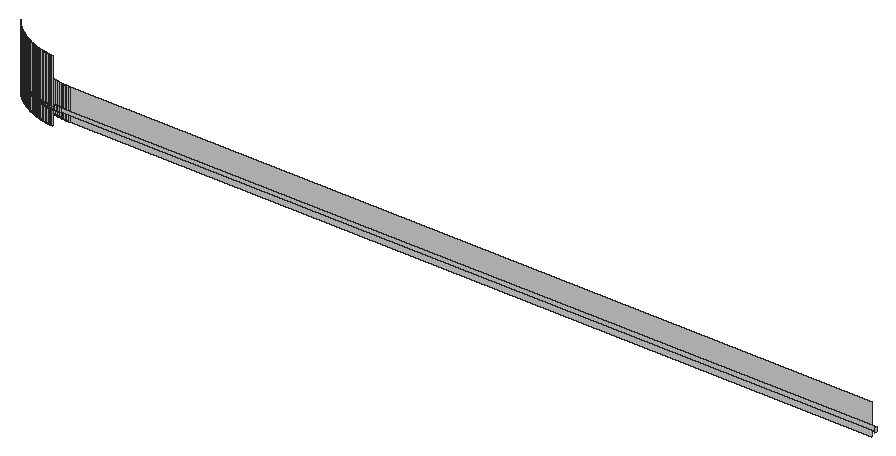
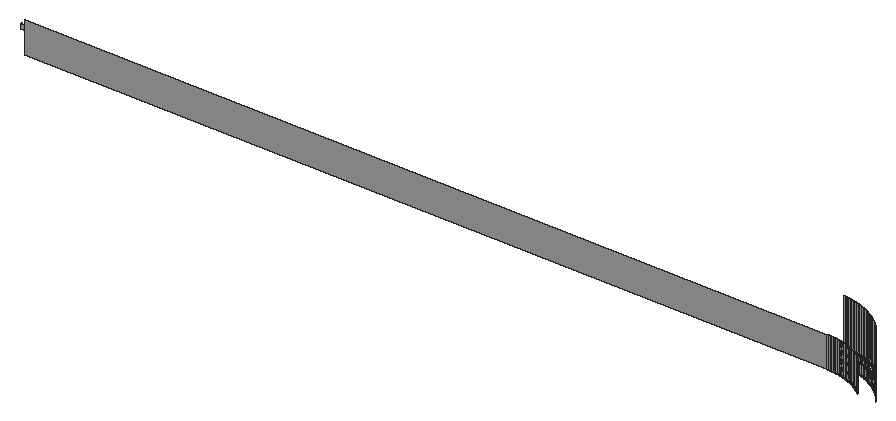
# SketchUp Ruby script. Lengths in inches.
U = 1.inch
M = Sketchup.active_model
def pt(a) = Geom::Point3d.new(a.map { |v| v * U })
def face(e, loops, mat)
  f = e.add_face(loops[0].map { |a| pt(a) })
  loops[1..].each { |l| e.add_face(l.map { |a| pt(a) }).erase! }
  f.material = f.back_material = mat if mat
  f
end
# faces: each face lists its corners as indices into pts; further lists are holes
def faces(e, pts, list, mat = nil) = list.each { |f| face(e, (f[0].is_a?(Array) ? f : [f]).map { |l| l.map { |i| pts[i] } }, mat) }
# xy, xz, yz: faces in a plane at the given z, y or x. An outline is a flat list of corners, or four numbers for a rectangle; further outlines are holes
def ring(l) = l.size == 4 ? [[l[0], l[1]], [l[2], l[1]], [l[2], l[3]], [l[0], l[3]]] : l.each_slice(2).to_a
def flat(e, list, mat, &to3) = list.each { |f| face(e, (f[0].is_a?(Array) ? f : [f]).map { |l| ring(l).map { |u, v| to3.(u, v) } }, mat) }
def xy(e, z, list, mat = nil) = flat(e, list, mat) { |x, y| [x, y, z] }
def xz(e, y, list, mat = nil) = flat(e, list, mat) { |x, z| [x, y, z] }
def yz(e, x, list, mat = nil) = flat(e, list, mat) { |y, z| [x, y, z] }
def lines(e, pts, list) = list.each { |a, b| e.add_line(pt(pts[a]), pt(pts[b])) }
# prism: a flat outline (further loops are holes) pulled along v
def prism(e, loops, v, mat = nil)
  f = face(e, loops, mat); d = Geom::Vector3d.new(v.map { |x| x * U })
  f.pushpull(f.normal.samedirection?(d) ? d.length : -d.length)
end
def box(e, o, s, mat = nil) = prism(e, [[o, [o[0] + s[0], o[1], o[2]], [o[0] + s[0], o[1] + s[1], o[2]], [o[0], o[1] + s[1], o[2]]]], [0, 0, s[2]], mat)
def at(x, y, z, deg = 0) = Geom::Transformation.translation(pt([x, y, z])) * Geom::Transformation.rotation(ORIGIN, Z_AXIS, deg.degrees)
def axes(o, x, y, z) = Geom::Transformation.new([*x, 0, *y, 0, *z, 0, *pt(o).to_a, 1])
def part(name) = M.definitions.add(name)
# library, detail: a bought-in or finely detailed component or shape, given as its bounding box
def library(name, o, s) = part(name).tap { |d| box(d.entities, o, s) }
def detail(e, o, s) = box(e.add_group.entities, o, s)
def put(e, d, t, mat = nil) = e.add_instance(d, t).tap { |i| i.material = mat if mat }
def group(e, t, mat = nil) = e.add_group.tap { |g| g.transformation = t; g.material = mat if mat }.entities
root = M.entities
M.materials.add("[Quartz Light Brown]").color = [215, 212, 212]
xz(root,194.5,[[17.77,114,18,115],[18,114,201,115]],"[Quartz Light Brown]")
xz(root,194.51,[[17.3125,114,17.54,115]],"[Quartz Light Brown]")
xz(root,197,[[17.8,111,18,118],[18,111,198,118]],"[Quartz Light Brown]")
xz(root,197.01,[[17.41,111,17.61,118]],"[Quartz Light Brown]")
yz(root,201,[[194,114,194.5,115]],"[Quartz Light Brown]")
p = [[15.65,194.15,114],[15.65,194.15,111],[15.88,194.125,111],[15.88,194.125,114],[16.12,194.1,111],[16.12,194.1,114],
  [16.35,194.08,111],[16.35,194.08,114],[16.59,194.06,111],[16.59,194.06,114],[14.95,194.26,114],[14.95,194.26,111],
  [15.18,194.22,111],[15.18,194.22,114],[15.42,194.1875,111],[15.42,194.1875,114],[14.26,194.39,114],[14.26,194.39,111],
  [14.49,194.35,111],[14.49,194.35,114],[14.72,194.3,111],[14.72,194.3,114],[13.8,194.5,114],[13.8,194.5,111],
  [14.03,194.44,111],[14.03,194.44,114],[13.57,194.55,114],[13.57,194.55,111],[13.11,194.68,114],[13.11,194.68,111],
  [13.34,194.61,111],[13.34,194.61,114],[12.66,194.81,114],[12.66,194.81,111],[12.89,194.74,111],[12.89,194.74,114],
  [12.4375,194.88,114],[12.4375,194.88,111],[12.21,194.96,114],[12.21,194.96,111],[11.77,195.11,114],[11.77,195.11,111],
  [11.99,195.03,111],[11.99,195.03,114],[11.55,195.2,114],[11.55,195.2,111],[11.33,195.28,114],[11.33,195.28,111],
  [11.11,195.37,114],[11.11,195.37,111],[10.89,195.46,114],[10.89,195.46,111],[10.68,195.56,114],[10.68,195.56,111],
  [10.46,195.65,114],[10.46,195.65,111],[10.25,195.75,114],[10.25,195.75,111],[10.04,195.86,114],[10.04,195.86,111],
  [9.83,195.96,114],[9.83,195.96,111],[9.62,196.07,114],[9.62,196.07,111],[9.41,196.18,114],[9.41,196.18,111],
  [9.2,196.3,114],[9.2,196.3,111],[9,196.41,114],[9,196.41,111],[8.8,196.53,114],[8.8,196.53,111],
  [8.6,196.65,114],[8.6,196.65,111],[8.39,196.78,114],[8.39,196.78,111],[8.2,196.9,114],[8.2,196.9,111],
  [8,197.03,114],[8,197.03,111],[7.8,197.17,114],[7.8,197.17,111],[16.63,197.0625,118],[16.82,197.05,118],
  [16.82,197.05,111],[16.63,197.0625,111],[17.02,197.03,118],[17.02,197.03,111],[17.21,197.02,118],[17.21,197.02,111],
  [17.41,197.01,118],[17.41,197.01,111],[17.61,197.01,118],[17.8,197,118],[17.8,197,111],[17.61,197.01,111],
  [15.85,197.16,118],[16.04,197.13,118],[16.04,197.13,111],[15.85,197.16,111],[16.24,197.1,118],[16.24,197.1,111],
  [16.43,197.08,118],[16.43,197.08,111],[7.61,197.3,114],[7.61,197.3,111],[15.27,197.25,118],[15.46,197.22,118],
  [15.46,197.22,111],[15.27,197.25,111],[15.65,197.18,118],[15.65,197.18,111],[7.42,197.4375,114],[7.42,197.4375,111],
  [14.69,197.37,118],[14.88,197.33,118],[14.88,197.33,111],[14.69,197.37,111],[15.07,197.29,118],[15.07,197.29,111],
  [7.23,197.58,114],[7.23,197.58,111],[14.31,197.46,118],[14.5,197.41,118],[14.5,197.41,111],[14.31,197.46,111],
  [13.93,197.5625,118],[14.12,197.51,118],[14.12,197.51,111],[13.93,197.5625,111],[7.04,197.72,114],[7.04,197.72,111],
  [13.55,197.67,118],[13.74,197.62,118],[13.74,197.62,111],[13.55,197.67,111],[6.86,197.86,114],[6.86,197.86,111],
  [13.18,197.8,118],[13.36,197.73,118],[13.36,197.73,111],[13.18,197.8,111],[12.99,197.86,118],[12.99,197.86,111],
  [6.67,198.01,114],[6.67,198.01,111],[12.625,198,118],[12.81,197.93,118],[12.81,197.93,111],[12.625,198,111],
  [6.49,198.16,114],[6.49,198.16,111],[12.44,198.07,118],[12.44,198.07,111],[12.08,198.22,118],[12.26,198.14,118],
  [12.26,198.14,111],[12.08,198.22,111],[6.31,198.3125,114],[6.31,198.3125,111],[11.9,198.3,118],[11.9,198.3,111],
  [6.13,198.47,114],[6.13,198.47,111],[11.72,198.38,118],[11.72,198.38,111],[11.54,198.46,118],[11.54,198.46,111],
  [5.96,198.625,114],[5.96,198.625,111],[11.19,198.63,118],[11.37,198.55,118],[11.37,198.55,111],[11.19,198.63,111],
  [5.78,198.78,114],[5.78,198.78,111],[11.02,198.73,118],[11.02,198.73,111],[10.84,198.82,118],[10.84,198.82,111],
  [5.61,198.94,114],[5.61,198.94,111],[10.67,198.91,118],[10.67,198.91,111],[5.44,199.11,114],[5.44,199.11,111],
  [10.5,199.01,118],[10.5,199.01,111],[10.33,199.11,118],[10.33,199.11,111],[5.27,199.27,114],[5.27,199.27,111],
  [10.16,199.21,118],[10.16,199.21,111],[10,199.3125,118],[10,199.3125,111],[5.11,199.44,114],[5.11,199.44,111],
  [9.83,199.42,118],[9.83,199.42,111],[4.94,199.61,114],[4.94,199.61,111],[9.67,199.53,118],[9.67,199.53,111],
  [9.5,199.64,118],[9.5,199.64,111],[4.78,199.78,114],[4.78,199.78,111],[9.34,199.75,118],[9.34,199.75,111],
  [4.625,199.96,114],[4.625,199.96,111],[9.18,199.86,118],[9.18,199.86,111],[9.03,199.98,118],[9.03,199.98,111],
  [4.47,200.13,114],[4.47,200.13,111],[8.87,200.1,118],[8.87,200.1,111],[4.3125,200.31,114],[4.3125,200.31,111],
  [8.71,200.22,118],[8.71,200.22,111],[8.56,200.34,118],[8.56,200.34,111],[4.16,200.49,114],[4.16,200.49,111],
  [8.41,200.47,118],[8.41,200.47,111],[4.01,200.67,114],[4.01,200.67,111],[8.26,200.59,118],[8.26,200.59,111],
  [16.625,194.55,115],[16.625,194.55,114],[16.86,194.54,114],[16.86,194.54,115],[17.08,194.52,114],[17.08,194.52,115],
  [17.3125,194.51,114],[17.3125,194.51,115],[17.54,194.51,115],[17.54,194.51,114],[17.77,194.5,114],[17.77,194.5,115],
  [15.49,194.68,115],[15.49,194.68,114],[15.72,194.65,114],[15.72,194.65,115],[15.94,194.62,114],[15.94,194.62,115],
  [16.17,194.6,114],[16.17,194.6,115],[16.4,194.57,114],[16.4,194.57,115],[15.04,194.75,115],[15.04,194.75,114],
  [15.26,194.72,114],[15.26,194.72,115],[14.36,194.88,115],[14.36,194.88,114],[14.59,194.84,114],[14.59,194.84,115],
  [14.8125,194.79,114],[14.8125,194.79,115],[13.91,194.98,115],[13.91,194.98,114],[14.14,194.93,114],[14.14,194.93,115],
  [13.47,195.1,115],[13.47,195.1,114],[13.69,195.04,114],[13.69,195.04,115],[13.25,195.16,115],[13.25,195.16,114],
  [12.8125,195.29,115],[12.8125,195.29,114],[13.03,195.22,114],[13.03,195.22,115],[12.59,195.36,115],[12.59,195.36,114],
  [12.16,195.5,115],[12.16,195.5,114],[12.375,195.43,114],[12.375,195.43,115],[11.94,195.58,115],[11.94,195.58,114],
  [11.73,195.66,115],[11.73,195.66,114],[11.3,195.83,115],[11.3,195.83,114],[11.52,195.75,114],[11.52,195.75,115],
  [11.09,195.92,115],[11.09,195.92,114],[10.88,196.01,115],[10.88,196.01,114],[10.67,196.11,115],[10.67,196.11,114],
  [10.47,196.2,115],[10.47,196.2,114],[10.26,196.3,115],[10.26,196.3,114],[10.06,196.41,115],[10.06,196.41,114],
  [9.85,196.51,115],[9.85,196.51,114],[9.65,196.62,115],[9.65,196.62,114],[9.45,196.73,115],[9.45,196.73,114],
  [9.25,196.84,115],[9.25,196.84,114],[9.05,196.96,115],[9.05,196.96,114],[8.86,197.08,115],[8.86,197.08,114],
  [8.66,197.2,115],[8.66,197.2,114],[8.47,197.32,115],[8.47,197.32,114],[8.28,197.45,115],[8.28,197.45,114],
  [8.09,197.58,115],[8.09,197.58,114],[7.9,197.71,115],[7.9,197.71,114],[7.71,197.84,115],[7.71,197.84,114],
  [7.53,197.98,115],[7.53,197.98,114],[7.35,198.12,115],[7.35,198.12,114],[7.17,198.26,115],[7.17,198.26,114],
  [6.99,198.4,115],[6.99,198.4,114],[6.81,198.55,115],[6.81,198.55,114],[6.63,198.69,115],[6.63,198.69,114],
  [6.46,198.84,115],[6.46,198.84,114],[6.29,198.99,115],[6.29,198.99,114],[6.12,199.15,115],[6.12,199.15,114],
  [5.95,199.31,115],[5.95,199.31,114],[5.79,199.46,115],[5.79,199.46,114],[5.625,199.625,115],[5.625,199.625,114],
  [5.46,199.79,115],[5.46,199.79,114],[5.31,199.95,115],[5.31,199.95,114],[5.15,200.12,115],[5.15,200.12,114],
  [4.99,200.29,115],[4.99,200.29,114],[4.84,200.46,115],[4.84,200.46,114],[4.69,200.63,115],[4.69,200.63,114],
  [15.65,194.15,125],[15.65,194.15,115],[15.88,194.125,115],[15.88,194.125,125],[16.12,194.1,115],[16.12,194.1,125],
  [16.35,194.08,115],[16.35,194.08,125],[16.59,194.06,115],[16.59,194.06,125],[14.95,194.26,125],[14.95,194.26,115],
  [15.18,194.22,115],[15.18,194.22,125],[15.42,194.1875,115],[15.42,194.1875,125],[14.26,194.39,125],[14.26,194.39,115],
  [14.49,194.35,115],[14.49,194.35,125],[14.72,194.3,115],[14.72,194.3,125],[13.8,194.5,125],[13.8,194.5,115],
  [14.03,194.44,115],[14.03,194.44,125],[13.57,194.55,125],[13.57,194.55,115],[13.11,194.68,125],[13.11,194.68,115],
  [13.34,194.61,115],[13.34,194.61,125],[12.66,194.81,125],[12.66,194.81,115],[12.89,194.74,115],[12.89,194.74,125],
  [12.4375,194.88,125],[12.4375,194.88,115],[12.21,194.96,125],[12.21,194.96,115],[11.77,195.11,125],[11.77,195.11,115],
  [11.99,195.03,115],[11.99,195.03,125],[11.55,195.2,125],[11.55,195.2,115],[11.33,195.28,125],[11.33,195.28,115],
  [11.11,195.37,125],[11.11,195.37,115],[10.89,195.46,125],[10.89,195.46,115],[10.68,195.56,125],[10.68,195.56,115],
  [10.46,195.65,125],[10.46,195.65,115],[10.25,195.75,125],[10.25,195.75,115],[10.04,195.86,125],[10.04,195.86,115],
  [9.83,195.96,125],[9.83,195.96,115],[9.62,196.07,125],[9.62,196.07,115],[9.41,196.18,125],[9.41,196.18,115],
  [9.2,196.3,125],[9.2,196.3,115],[9,196.41,125],[9,196.41,115],[8.8,196.53,125],[8.8,196.53,115],
  [8.6,196.65,125],[8.6,196.65,115],[8.39,196.78,125],[8.39,196.78,115],[8.2,196.9,125],[8.2,196.9,115],
  [8,197.03,125],[8,197.03,115],[7.8,197.17,125],[7.8,197.17,115],[7.61,197.3,125],[7.61,197.3,115],
  [7.42,197.4375,125],[7.42,197.4375,115],[7.23,197.58,125],[7.23,197.58,115],[7.04,197.72,125],[7.04,197.72,115],
  [6.86,197.86,125],[6.86,197.86,115],[6.67,198.01,125],[6.67,198.01,115],[6.49,198.16,125],[6.49,198.16,115],
  [6.31,198.3125,125],[6.31,198.3125,115],[6.13,198.47,125],[6.13,198.47,115],[5.96,198.625,125],[5.96,198.625,115],
  [5.78,198.78,125],[5.78,198.78,115],[5.61,198.94,125],[5.61,198.94,115],[5.44,199.11,125],[5.44,199.11,115],
  [5.27,199.27,125],[5.27,199.27,115],[5.11,199.44,125],[5.11,199.44,115],[4.94,199.61,125],[4.94,199.61,115],
  [4.78,199.78,125],[4.78,199.78,115],[4.625,199.96,125],[4.625,199.96,115],[4.47,200.13,125],[4.47,200.13,115],
  [4.3125,200.31,125],[4.3125,200.31,115],[4.16,200.49,125],[4.16,200.49,115]]
faces(root,p,[[0,1,2,3],[3,2,4,5],[5,4,6,7],[7,6,8,9],[10,11,12,13],[13,12,14,15],[15,14,1,0],[16,17,18,19],
  [19,18,20,21],[21,20,11,10],[22,23,24,25],[25,24,17,16],[26,27,23,22],[28,29,30,31],[31,30,27,26],[32,33,34,35],
  [35,34,29,28],[36,37,33,32],[38,39,37,36],[40,41,42,43],[43,42,39,38],[44,45,41,40],[46,47,45,44],[48,49,47,46],
  [50,51,49,48],[52,53,51,50],[54,55,53,52],[56,57,55,54],[58,59,57,56],[60,61,59,58],[62,63,61,60],[64,65,63,62],
  [66,67,65,64],[68,69,67,66],[70,71,69,68],[72,73,71,70],[74,75,73,72],[76,77,75,74],[78,79,77,76],[80,81,79,78],
  [82,83,84,85],[83,86,87,84],[86,88,89,87],[88,90,91,89],[92,93,94,95],[96,97,98,99],[97,100,101,98],[100,102,103,101],
  [102,82,85,103],[104,105,81,80],[106,107,108,109],[107,110,111,108],[110,96,99,111],[112,113,105,104],[114,115,116,117],[115,118,119,116],
  [118,106,109,119],[120,121,113,112],[122,123,124,125],[123,114,117,124],[126,127,128,129],[127,122,125,128],[130,131,121,120],[132,133,134,135],
  [133,126,129,134],[136,137,131,130],[138,139,140,141],[139,132,135,140],[142,138,141,143],[144,145,137,136],[146,147,148,149],[147,142,143,148],
  [150,151,145,144],[152,146,149,153],[154,155,156,157],[155,152,153,156],[158,159,151,150],[160,154,157,161],[162,163,159,158],[164,160,161,165],
  [166,164,165,167],[168,169,163,162],[170,171,172,173],[171,166,167,172],[174,175,169,168],[176,170,173,177],[178,176,177,179],[180,181,175,174],
  [182,178,179,183],[184,185,181,180],[186,182,183,187],[188,186,187,189],[190,191,185,184],[192,188,189,193],[194,192,193,195],[196,197,191,190],
  [198,194,195,199],[200,201,197,196],[202,198,199,203],[204,202,203,205],[206,207,201,200],[208,204,205,209],[210,211,207,206],[212,208,209,213],
  [214,212,213,215],[216,217,211,210],[218,214,215,219],[220,221,217,216],[222,218,219,223],[224,222,223,225],[226,227,221,220],[228,224,225,229],
  [230,231,227,226],[232,228,229,233],[234,235,236,237],[237,236,238,239],[239,238,240,241],[242,243,244,245],[246,247,248,249],[249,248,250,251],
  [251,250,252,253],[253,252,254,255],[255,254,235,234],[256,257,258,259],[259,258,247,246],[260,261,262,263],[263,262,264,265],[265,264,257,256],
  [266,267,268,269],[269,268,261,260],[270,271,272,273],[273,272,267,266],[274,275,271,270],[276,277,278,279],[279,278,275,274],[280,281,277,276],
  [282,283,284,285],[285,284,281,280],[286,287,283,282],[288,289,287,286],[290,291,292,293],[293,292,289,288],[294,295,291,290],[296,297,295,294],
  [298,299,297,296],[300,301,299,298],[302,303,301,300],[304,305,303,302],[306,307,305,304],[308,309,307,306],[310,311,309,308],[312,313,311,310],
  [314,315,313,312],[316,317,315,314],[318,319,317,316],[320,321,319,318],[322,323,321,320],[324,325,323,322],[326,327,325,324],[328,329,327,326],
  [330,331,329,328],[332,333,331,330],[334,335,333,332],[336,337,335,334],[338,339,337,336],[340,341,339,338],[342,343,341,340],[344,345,343,342],
  [346,347,345,344],[348,349,347,346],[350,351,349,348],[352,353,351,350],[354,355,353,352],[356,357,355,354],[358,359,357,356],[360,361,359,358],
  [362,363,361,360],[364,365,363,362],[366,367,368,369],[369,368,370,371],[371,370,372,373],[373,372,374,375],[376,377,378,379],[379,378,380,381],
  [381,380,367,366],[382,383,384,385],[385,384,386,387],[387,386,377,376],[388,389,390,391],[391,390,383,382],[392,393,389,388],[394,395,396,397],
  [397,396,393,392],[398,399,400,401],[401,400,395,394],[402,403,399,398],[404,405,403,402],[406,407,408,409],[409,408,405,404],[410,411,407,406],
  [412,413,411,410],[414,415,413,412],[416,417,415,414],[418,419,417,416],[420,421,419,418],[422,423,421,420],[424,425,423,422],[426,427,425,424],
  [428,429,427,426],[430,431,429,428],[432,433,431,430],[434,435,433,432],[436,437,435,434],[438,439,437,436],[440,441,439,438],[442,443,441,440],
  [444,445,443,442],[446,447,445,444],[448,449,447,446],[450,451,449,448],[452,453,451,450],[454,455,453,452],[456,457,455,454],[458,459,457,456],
  [460,461,459,458],[462,463,461,460],[464,465,463,462],[466,467,465,464],[468,469,467,466],[470,471,469,468],[472,473,471,470],[474,475,473,472],
  [476,477,475,474],[478,479,477,476],[480,481,479,478],[482,483,481,480],[484,485,483,482],[486,487,485,484],[488,489,487,486]],"[Quartz Light Brown]")
